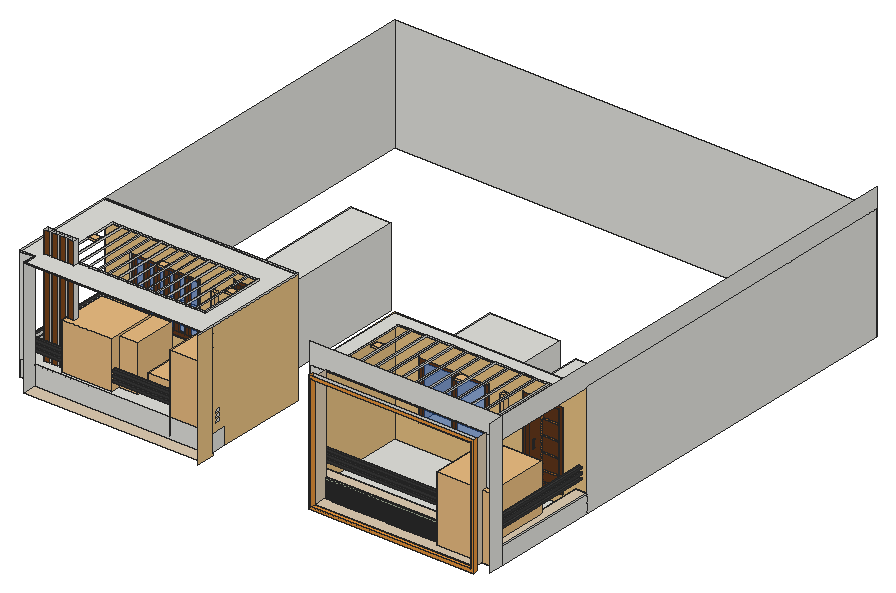
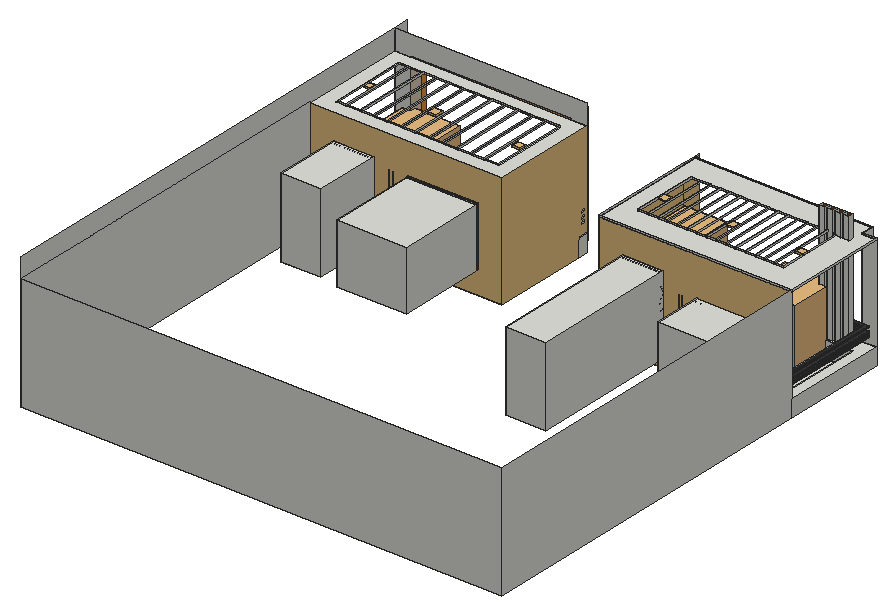
# SketchUp Ruby script. Lengths in inches.
U = 1.inch
M = Sketchup.active_model
def pt(a) = Geom::Point3d.new(a.map { |v| v * U })
def face(e, loops, mat)
  f = e.add_face(loops[0].map { |a| pt(a) })
  loops[1..].each { |l| e.add_face(l.map { |a| pt(a) }).erase! }
  f.material = f.back_material = mat if mat
  f
end
# faces: each face lists its corners as indices into pts; further lists are holes
def faces(e, pts, list, mat = nil) = list.each { |f| face(e, (f[0].is_a?(Array) ? f : [f]).map { |l| l.map { |i| pts[i] } }, mat) }
# xy, xz, yz: faces in a plane at the given z, y or x. An outline is a flat list of corners, or four numbers for a rectangle; further outlines are holes
def ring(l) = l.size == 4 ? [[l[0], l[1]], [l[2], l[1]], [l[2], l[3]], [l[0], l[3]]] : l.each_slice(2).to_a
def flat(e, list, mat, &to3) = list.each { |f| face(e, (f[0].is_a?(Array) ? f : [f]).map { |l| ring(l).map { |u, v| to3.(u, v) } }, mat) }
def xy(e, z, list, mat = nil) = flat(e, list, mat) { |x, y| [x, y, z] }
def xz(e, y, list, mat = nil) = flat(e, list, mat) { |x, z| [x, y, z] }
def yz(e, x, list, mat = nil) = flat(e, list, mat) { |y, z| [x, y, z] }
def lines(e, pts, list) = list.each { |a, b| e.add_line(pt(pts[a]), pt(pts[b])) }
# prism: a flat outline (further loops are holes) pulled along v
def prism(e, loops, v, mat = nil)
  f = face(e, loops, mat); d = Geom::Vector3d.new(v.map { |x| x * U })
  f.pushpull(f.normal.samedirection?(d) ? d.length : -d.length)
end
def box(e, o, s, mat = nil) = prism(e, [[o, [o[0] + s[0], o[1], o[2]], [o[0] + s[0], o[1] + s[1], o[2]], [o[0], o[1] + s[1], o[2]]]], [0, 0, s[2]], mat)
def at(x, y, z, deg = 0) = Geom::Transformation.translation(pt([x, y, z])) * Geom::Transformation.rotation(ORIGIN, Z_AXIS, deg.degrees)
def axes(o, x, y, z) = Geom::Transformation.new([*x, 0, *y, 0, *z, 0, *pt(o).to_a, 1])
def part(name) = M.definitions.add(name)
# library, detail: a bought-in or finely detailed component or shape, given as its bounding box
def library(name, o, s) = part(name).tap { |d| box(d.entities, o, s) }
def detail(e, o, s) = box(e.add_group.entities, o, s)
def put(e, d, t, mat = nil) = e.add_instance(d, t).tap { |i| i.material = mat if mat }
def group(e, t, mat = nil) = e.add_group.tap { |g| g.transformation = t; g.material = mat if mat }.entities
root = M.entities
M.materials.add("Generic\#1").color = [121, 68, 27]
M.materials.add("Generic\#4").color = [232, 149, 60]
M.materials.add("Generic\#5").color = [233, 194, 132]
M.materials.add("Generic\#6").color = [223, 205, 179]
M.materials.add("Generic\#8").color = [168, 180, 155]
M.materials.add("[Color M05]").color = [114, 114, 114]
M.materials.add("[Color M07]").color = [58, 58, 58]
M.materials.add("[Translucent Glass Blue]").color = [28, 83, 181]
M.materials["[Translucent Glass Blue]"].alpha = 0.5
M.materials.add("[Wood Bamboo]").color = [177, 105, 43]
M.materials.add("[Wood Cherry Original]").color = [96, 54, 26]
c1 = library("Plante 4",[-1.67,-6.5,0],[37.31,31.95,64.42])
c2 = library("Group_2",[-1.28,-0.39,0],[21.22,20.51,48.44])
c3 = library("Group3\#1",[-238.15,54.18,0],[46.4,43.96,56.68])
c4 = library("Plant",[-27.84,-31.84,-1.26],[68.28,70.82,154.38])
c5 = library("Raised potted plant",[1.65,0,0],[13.63,13.63,20.73])
c6 = library("Plant+2 (1)",[-9.13,-9.52,0],[51.76,51.77,66.88])
c7 = part("Group\#12")
xy(c7.entities,17.5625,[[0,0,2,2]])
xz(c7.entities,0,[[0,0,2,17.5625]])
yz(c7.entities,0,[[0,0,2,17.5625]])
yz(c7.entities,2,[[0,0,2,17.5625]])
c8 = part("Group\#5")
xy(c8.entities,0,[[0,0,41.8125,3.4375]],"[Wood Cherry Original]")
xy(c8.entities,3.53,[[3.53,0,38.28,3.4375]],"[Wood Cherry Original]")
xy(c8.entities,31.39,[[9.28,1.32,9.97,3.4375]])
xy(c8.entities,32.05,[[9.29,1.98,9.98,3.4375]],"[Color M05]")
xy(c8.entities,39.77,[[9.29,1.98,9.98,3.4375]])
xy(c8.entities,40.43,[[9.28,1.32,9.97,3.4375]],"[Color M05]")
xy(c8.entities,79.47,[[3.53,0,38.28,3.4375]],"[Wood Cherry Original]")
xy(c8.entities,83,[[0,0,41.8125,3.4375]],"[Wood Cherry Original]")
xz(c8.entities,0,[[[0,0,41.8125,83],[3.53,3.53,38.28,79.47]]],"[Wood Cherry Original]")
xz(c8.entities,1.32,[[9.28,31.39,9.97,40.43]],"[Color M05]")
xz(c8.entities,1.98,[[9.29,32.05,9.98,39.77]],"[Color M05]")
xz(c8.entities,3.4375,[[9.29,39.77,9.28,40.43,9.97,40.43,9.98,39.77]])
xz(c8.entities,3.4375,[[16.22,3.53,17.74,3.53,17.74,13.29,38.28,13.29,38.28,15.09,17.74,15.09,17.74,29.41,38.28,29.41,38.28,31.22,17.74,31.22,17.74,45.54,38.28,45.54,38.28,47.34,17.74,47.34,17.74,61.66,38.28,61.66,38.28,63.47,17.74,63.47,17.74,79.47,16.22,79.47]],"[Wood Bamboo]")
xz(c8.entities,3.4375,[[[0,0,41.8125,83],[3.53,3.53,38.28,79.47]],[[3.53,3.53,16.22,79.47],[9.29,39.77,9.28,40.43,9.97,40.43,9.98,39.77],[9.28,31.39,9.29,32.05,9.98,32.05,9.97,31.39]],[17.74,3.53,38.28,13.29],[17.74,15.09,38.28,29.41],[17.74,31.22,38.28,45.54],
  [17.74,47.34,38.28,61.66],[17.74,63.47,38.28,79.47]],"[Wood Cherry Original]")
yz(c8.entities,0,[[0,0,3.4375,83]],"[Wood Cherry Original]")
yz(c8.entities,3.53,[[0,3.53,3.4375,79.47]],"[Wood Cherry Original]")
yz(c8.entities,38.28,[[0,3.53,3.4375,79.47]],"[Wood Cherry Original]")
yz(c8.entities,41.8125,[[0,0,3.4375,83]],"[Wood Cherry Original]")
p = [[9.28,1.32,40.43],[9.29,1.98,39.77],[9.29,1.98,32.05],[9.28,1.32,31.39],[9.29,3.4375,32.05],[9.28,3.4375,31.39],
  [9.98,1.98,39.77],[9.97,1.32,40.43],[9.97,1.32,31.39],[9.98,1.98,32.05],[9.97,3.4375,31.39],[9.98,3.4375,32.05],
  [9.28,3.4375,40.43],[9.29,3.4375,39.77],[9.98,3.4375,39.77],[9.97,3.4375,40.43],[9.625,3.4375,40.13],[9.625,1.625,40.13],
  [9.625,1.625,31.69],[9.625,3.4375,31.69]]
faces(c8.entities,p,[[0,1,2,3],[3,2,4,5],[6,7,8,9],[9,8,10,11],[12,13,1,0],[14,15,7,6]],"[Color M05]")
lines(c8.entities,p,[[16,17],[18,19],[17,18]])
c9 = part("Group\#3")
xy(c9.entities,0,[[0,0,81.86,2.5]],"[Wood Cherry Original]")
xy(c9.entities,4.12,[[4.12,0,13.68,2.5],[13.68,0,18.93,2.5],[18.93,0,25.68,2.5],[25.68,0,30.93,2.5],[30.93,0,37.68,2.5],
  [37.68,0,42.93,2.5],[42.93,0,49.68,2.5],[49.68,0,54.93,2.5],[54.93,0,61.68,2.5],[61.68,0,66.93,2.5],
  [66.93,0,77.74,2.5]],"[Wood Cherry Original]")
xy(c9.entities,66.49,[[4.12,0,13.68,2.5],[13.68,0,18.93,2.5],[18.93,0,25.68,2.5],[25.68,0,30.93,2.5],[30.93,0,37.68,2.5],
  [37.68,0,42.93,2.5],[42.93,0,49.68,2.5],[49.68,0,54.93,2.5],[54.93,0,61.68,2.5],[61.68,0,66.93,2.5],
  [66.93,0,77.74,2.5]],"[Wood Cherry Original]")
xy(c9.entities,70.61,[[0,0,81.86,2.5]],"[Wood Cherry Original]")
xz(c9.entities,0,[[[0,0,81.86,70.61],[4.12,4.12,77.74,66.49]],[13.68,4.12,18.93,66.49],[25.68,4.12,30.93,66.49],[37.68,4.12,42.93,66.49],[49.68,4.12,54.93,66.49],
  [61.68,4.12,66.93,66.49]],"[Wood Cherry Original]")
xz(c9.entities,2.5,[[4.12,4.12,13.68,66.49],[18.93,4.12,25.68,66.49],[30.93,4.12,37.68,66.49],[42.93,4.12,49.68,66.49],[54.93,4.12,61.68,66.49],
  [66.93,4.12,77.74,66.49]],"[Translucent Glass Blue]")
xz(c9.entities,2.5,[[[0,0,81.86,70.61],[4.12,4.12,77.74,66.49]]],"[Wood Cherry Original]")
yz(c9.entities,0,[[0,0,2.5,70.61]],"[Wood Cherry Original]")
yz(c9.entities,4.12,[[0,4.12,2.5,66.49]],"[Wood Cherry Original]")
yz(c9.entities,13.68,[[0,4.12,2.5,66.49]],"[Wood Cherry Original]")
yz(c9.entities,18.93,[[0,4.12,2.5,66.49]],"[Wood Cherry Original]")
yz(c9.entities,25.68,[[0,4.12,2.5,66.49]],"[Wood Cherry Original]")
yz(c9.entities,30.93,[[0,4.12,2.5,66.49]],"[Wood Cherry Original]")
yz(c9.entities,37.68,[[0,4.12,2.5,66.49]],"[Wood Cherry Original]")
yz(c9.entities,42.93,[[0,4.12,2.5,66.49]],"[Wood Cherry Original]")
yz(c9.entities,49.68,[[0,4.12,2.5,66.49]],"[Wood Cherry Original]")
yz(c9.entities,54.93,[[0,4.12,2.5,66.49]],"[Wood Cherry Original]")
yz(c9.entities,61.68,[[0,4.12,2.5,66.49]],"[Wood Cherry Original]")
yz(c9.entities,66.93,[[0,4.12,2.5,66.49]],"[Wood Cherry Original]")
yz(c9.entities,77.74,[[0,4.12,2.5,66.49]],"[Wood Cherry Original]")
yz(c9.entities,81.86,[[0,0,2.5,70.61]],"[Wood Cherry Original]")
c10 = part("Group\#4")
xy(c10.entities,0,[[0,0,73.625,2.0625]],"[Wood Cherry Original]")
xy(c10.entities,3.98,[[35.0625,0,38.75,2.0625]])
xy(c10.entities,3.98,[[3.98,0,35.0625,2.0625],[38.75,0,69.64,2.0625]],"[Wood Cherry Original]")
xy(c10.entities,58.39,[[35.0625,0,38.75,2.0625]])
xy(c10.entities,58.39,[[3.98,0,35.0625,2.0625],[38.75,0,69.64,2.0625]],"[Wood Cherry Original]")
xy(c10.entities,62.375,[[0,0,73.625,2.0625]],"[Wood Cherry Original]")
xz(c10.entities,0,[[[0,0,73.625,62.375],[3.98,3.98,69.64,58.39]],[35.0625,3.98,38.75,58.39]],"[Wood Cherry Original]")
xz(c10.entities,2.0625,[[[0,0,73.625,62.375],[3.98,3.98,69.64,58.39]]])
xz(c10.entities,2.0625,[[3.98,3.98,35.0625,58.39],[38.75,3.98,69.64,58.39]],"[Translucent Glass Blue]")
yz(c10.entities,0,[[0,0,2.0625,62.375]],"[Wood Cherry Original]")
yz(c10.entities,3.98,[[0,3.98,2.0625,58.39]],"[Wood Cherry Original]")
yz(c10.entities,35.0625,[[0,3.98,2.0625,58.39]],"[Wood Cherry Original]")
yz(c10.entities,38.75,[[0,3.98,2.0625,58.39]],"[Wood Cherry Original]")
yz(c10.entities,69.64,[[0,3.98,2.0625,58.39]],"[Wood Cherry Original]")
yz(c10.entities,73.625,[[0,0,2.0625,62.375]],"[Wood Cherry Original]")
c11 = library("Lamp Wall Outdoor 94-02",[-1.89,-4.65,-3.17],[3.78,4.65,6.35])
c12 = library("Tlon Light 450 Ceiling 152 006",[-8.86,-8.86,-3.78],[17.72,17.72,3.56])
xy(root,278.625,[[321.31,34.75,494.1875,39.375]],"Generic\#4")
xy(root,278.75,[[17.125,41,204.09,54.5625]],"Generic\#6")
xy(root,281.75,[[306.09,54.5625,306.09,65.5625,496.1875,65.5625,496.1875,166.1875,507.875,166.1875,507.875,54.5625],[306.09,65.5625,496.1875,166.1875],[13.4375,71.3125,204.09,166.1875]])
xy(root,281.75,[[323.78,34.75,491.8125,39.375]],"Generic\#4")
xy(root,281.75,[[323.78,39.375,491.8125,54.5625]],"Generic\#6")
xy(root,289.8,[[137.36,166.1875,179.17,320.375]])
xy(root,290.68,[[440.99,166.1875,482.8,235.75]])
xy(root,297.03,[[27.78,166.1875,101.4,217.3125]])
xy(root,299.3125,[[323.78,52.5625,325.78,54.5625],[325.78,52.5625,491.8125,54.5625],[[2.3125,54.5625,204.09,54.5625,204.09,71.3125,13.4375,71.3125,13.4375,166.1875,2.3125,166.1875],[19.41,64.07,25.6,69.2],[27.85,64.07,34.03,69.2],[36.28,64.07,42.47,69.2],[44.72,64.07,50.91,69.2]],[306.09,54.5625,306.09,65.5625,496.1875,65.5625,496.1875,166.1875,507.875,166.1875,507.875,54.5625]])
xy(root,301.3125,[[306.09,54.5625,507.875,54.5625,507.875,166.1875,496.1875,166.1875,496.1875,65.5625,306.09,65.5625]],"Generic\#6")
xy(root,301.3125,[[323.78,52.5625,491.8125,54.5625]],"Generic\#8")
xy(root,305.15,[[331.4,166.1875,405.03,260.1875]])
xy(root,308.18,[[6.99,59.18,6.99,166.1875,10.24,166.1875,10.24,62.43,204.09,62.43,204.09,59.18]],"[Color M07]")
xy(root,310.93,[[6.99,59.18,204.09,59.18,204.09,62.43,10.24,62.43,10.24,166.1875,6.99,166.1875]],"[Color M07]")
xy(root,311.86,[[306.09,58.82,306.09,61.82,500.27,61.82,500.27,166.1875,503.27,166.1875,503.27,58.82]],"[Color M07]")
xy(root,312.62,[[6.99,59.18,6.99,166.1875,10.24,166.1875,10.24,62.43,204.09,62.43,204.09,59.18]],"[Color M07]")
xy(root,314.42,[[306.09,58.82,503.27,58.82,503.27,166.1875,500.27,166.1875,500.27,61.82,306.09,61.82]],"[Color M07]")
xy(root,315.37,[[6.99,59.18,204.09,59.18,204.09,62.43,10.24,62.43,10.24,166.1875,6.99,166.1875]],"[Color M07]")
xy(root,316.8,[[306.09,58.82,306.09,61.82,500.27,61.82,500.27,166.1875,503.27,166.1875,503.27,58.82]],"[Color M07]")
xy(root,317.37,[[6.99,59.18,6.99,166.1875,10.24,166.1875,10.24,62.43,204.09,62.43,204.09,59.18]],"[Color M07]")
xy(root,319.36,[[306.09,58.82,503.27,58.82,503.27,166.1875,500.27,166.1875,500.27,61.82,306.09,61.82]],"[Color M07]")
xy(root,320.12,[[6.99,59.18,204.09,59.18,204.09,62.43,10.24,62.43,10.24,166.1875,6.99,166.1875]],"[Color M07]")
xy(root,322.36,[[306.09,58.82,306.09,61.82,500.27,61.82,500.27,166.1875,503.27,166.1875,503.27,58.82]],"[Color M07]")
xy(root,324.92,[[306.09,58.82,503.27,58.82,503.27,166.1875,500.27,166.1875,500.27,61.82,306.09,61.82]],"[Color M07]")
xy(root,359.4,[[27.78,166.1875,101.4,217.3125]])
xy(root,367.53,[[331.4,166.1875,405.03,260.1875]])
xy(root,372.8,[[137.36,166.1875,179.17,320.375]])
xy(root,373.68,[[440.99,166.1875,482.8,235.75]])
xy(root,400.3125,[[[17.125,41,17.125,54.5625,2.3125,54.5625,2.3125,166.1875,204.09,166.1875,204.09,41],[32.72,68.9375,185.53,138.25]],[41.97,68.9375,42.91,138.25],[52.16,68.9375,53.09,138.25],[62.34,68.9375,63.28,138.25],[72.53,68.9375,73.47,138.25],
  [82.72,68.9375,83.66,138.25],[92.91,68.9375,93.84,138.25],[103.09,68.9375,104.03,138.25],[113.28,68.9375,114.22,138.25],[123.47,68.9375,124.41,138.25],
  [133.66,68.9375,134.59,138.25],[143.84,68.9375,144.78,138.25],[154.03,68.9375,154.97,138.25],[164.22,68.9375,165.16,138.25],[174.41,68.9375,175.34,138.25],
  [184.59,68.9375,185.53,138.25]])
xy(root,400.625,[[[306.09,54.5625,507.875,166.1875],[321.03,69.49,492.94,151.25]],[321.03,69.49,323.03,151.25],[335.53,69.49,337.53,151.25],[350.03,69.49,352.03,151.25],[364.53,69.49,366.53,151.25],
  [379.03,69.49,381.03,151.25],[393.53,69.49,395.53,151.25],[408.03,69.49,410.03,151.25],[422.53,69.49,424.53,151.25],[437.03,69.49,439.03,151.25],
  [451.53,69.49,453.53,151.25],[466.03,69.49,468.03,151.25],[480.53,69.49,482.53,151.25],[490.94,69.49,492.94,151.25]])
xz(root,34.75,[[[321.31,278.625,494.1875,404.6875],[323.78,281.75,491.8125,401.75]]],"Generic\#4")
xz(root,39.375,[[[321.31,278.625,494.1875,404.6875],[323.78,281.75,491.8125,401.75]]])
xz(root,41,[[17.125,400.3125,204.09,401.75]],"Generic\#4")
xz(root,52.5625,[[323.78,299.3125,491.8125,301.3125]],"Generic\#8")
xz(root,54.5625,[[17.125,278.75,204.09,299.3125],[2.3125,281.75,17.125,299.3125],[306.09,281.75,323.78,299.3125],[323.78,281.75,325.78,299.3125],[325.78,281.75,491.8125,299.3125],
  [491.8125,281.75,507.875,299.3125],[2.3125,299.3125,17.125,400.3125],[306.09,299.3125,323.78,301.3125],[323.78,299.3125,491.8125,301.3125],[491.8125,299.3125,507.875,301.3125],
  [306.09,301.3125,323.78,400.625],[491.8125,301.3125,507.875,400.625],[2.3125,400.3125,17.125,401.75],[306.09,400.625,306.09,422.625,507.875,422.625,507.875,400.625,491.8125,400.625,491.8125,401.75,323.78,401.75,323.78,400.625]])
xz(root,54.5625,[[323.78,400.625,491.8125,401.75]],"Generic\#4")
xz(root,58.82,[[306.09,311.86,503.27,314.42],[306.09,316.8,503.27,319.36],[306.09,322.36,503.27,324.92]],"[Color M07]")
xz(root,59.18,[[6.99,308.18,204.09,310.93],[6.99,312.62,204.09,315.37],[6.99,317.37,204.09,320.12]],"[Color M07]")
xz(root,61.82,[[306.09,311.86,500.27,314.42],[306.09,316.8,500.27,319.36],[306.09,322.36,500.27,324.92]],"[Color M07]")
xz(root,62.43,[[10.24,308.18,204.09,310.93],[10.24,312.62,204.09,315.37],[10.24,317.37,204.09,320.12]],"[Color M07]")
xz(root,64.07,[[19.41,299.3125,25.6,422.625],[27.85,299.3125,34.03,422.625],[36.28,299.3125,42.47,422.625],[44.72,299.3125,50.91,422.625]],"Generic\#1")
xz(root,65.5625,[[306.09,281.75,496.1875,299.3125],[306.09,299.3125,496.1875,301.3125]])
xz(root,68.9375,[[32.72,400.3125,41.97,401.75],[41.97,400.3125,42.91,401.75],[42.91,400.3125,52.16,401.75],[52.16,400.3125,53.09,401.75],[53.09,400.3125,62.34,401.75],
  [62.34,400.3125,63.28,401.75],[63.28,400.3125,72.53,401.75],[72.53,400.3125,73.47,401.75],[73.47,400.3125,82.72,401.75],[82.72,400.3125,83.66,401.75],
  [83.66,400.3125,92.91,401.75],[92.91,400.3125,93.84,401.75],[93.84,400.3125,103.09,401.75],[103.09,400.3125,104.03,401.75],[104.03,400.3125,113.28,401.75],
  [113.28,400.3125,114.22,401.75],[114.22,400.3125,123.47,401.75],[123.47,400.3125,124.41,401.75],[124.41,400.3125,133.66,401.75],[133.66,400.3125,134.59,401.75],
  [134.59,400.3125,143.84,401.75],[143.84,400.3125,144.78,401.75],[144.78,400.3125,154.03,401.75],[154.03,400.3125,154.97,401.75],[154.97,400.3125,164.22,401.75],
  [164.22,400.3125,165.16,401.75],[165.16,400.3125,174.41,401.75],[174.41,400.3125,175.34,401.75],[175.34,400.3125,184.59,401.75],[184.59,400.3125,185.53,401.75]])
xz(root,69.2,[[19.41,299.3125,25.6,422.625],[27.85,299.3125,34.03,422.625],[36.28,299.3125,42.47,422.625],[44.72,299.3125,50.91,422.625]])
xz(root,69.49,[[323.03,400.625,323.78,401.75],[323.78,400.625,335.53,401.75],[337.53,400.625,350.03,401.75],[352.03,400.625,364.53,401.75],[366.53,400.625,379.03,401.75],
  [381.03,400.625,393.53,401.75],[395.53,400.625,408.03,401.75],[410.03,400.625,422.53,401.75],[424.53,400.625,437.03,401.75],[439.03,400.625,451.53,401.75],
  [453.53,400.625,466.03,401.75],[468.03,400.625,480.53,401.75],[482.53,400.625,490.94,401.75]])
xz(root,71.3125,[[13.4375,281.75,204.09,299.3125]])
xz(root,138.25,[[32.72,400.3125,41.97,401.75],[41.97,400.3125,42.91,401.75],[42.91,400.3125,52.16,401.75],[52.16,400.3125,53.09,401.75],[53.09,400.3125,62.34,401.75],
  [62.34,400.3125,63.28,401.75],[63.28,400.3125,72.53,401.75],[72.53,400.3125,73.47,401.75],[73.47,400.3125,82.72,401.75],[82.72,400.3125,83.66,401.75],
  [83.66,400.3125,92.91,401.75],[92.91,400.3125,93.84,401.75],[93.84,400.3125,103.09,401.75],[103.09,400.3125,104.03,401.75],[104.03,400.3125,113.28,401.75],
  [113.28,400.3125,114.22,401.75],[114.22,400.3125,123.47,401.75],[123.47,400.3125,124.41,401.75],[124.41,400.3125,133.66,401.75],[133.66,400.3125,134.59,401.75],
  [134.59,400.3125,143.84,401.75],[143.84,400.3125,144.78,401.75],[144.78,400.3125,154.03,401.75],[154.03,400.3125,154.97,401.75],[154.97,400.3125,164.22,401.75],
  [164.22,400.3125,165.16,401.75],[165.16,400.3125,174.41,401.75],[174.41,400.3125,175.34,401.75],[175.34,400.3125,184.59,401.75],[184.59,400.3125,185.53,401.75]])
xz(root,151.25,[[323.03,400.625,335.53,401.75],[337.53,400.625,350.03,401.75],[352.03,400.625,364.53,401.75],[366.53,400.625,379.03,401.75],[381.03,400.625,393.53,401.75],
  [395.53,400.625,408.03,401.75],[410.03,400.625,422.53,401.75],[424.53,400.625,437.03,401.75],[439.03,400.625,451.53,401.75],[453.53,400.625,466.03,401.75],
  [468.03,400.625,480.53,401.75],[482.53,400.625,490.94,401.75]])
xz(root,166.1875,[[496.1875,299.3125,507.875,301.3125],[2.3125,400.3125,204.09,401.75]])
xz(root,166.1875,[[[13.4375,281.75,204.09,281.75,204.09,400.3125,2.3125,400.3125,2.3125,299.3125,13.4375,299.3125],[27.78,297.03,101.4,359.4],[137.36,289.8,179.17,372.8],[6.99,317.37,10.24,320.12],[6.99,312.62,10.24,315.37],[6.99,308.18,10.24,310.93]],[[306.09,281.75,496.1875,281.75,496.1875,301.3125,507.875,301.3125,507.875,400.625,306.09,400.625],[331.4,305.15,405.03,367.53],[440.99,290.68,482.8,373.68],[500.27,311.86,503.27,314.42],[500.27,316.8,503.27,319.36],[500.27,322.36,503.27,324.92]]],"Generic\#5")
xz(root,217.3125,[[27.78,297.03,101.4,359.4]])
xz(root,235.75,[[440.99,290.68,482.8,373.68]])
xz(root,260.1875,[[331.4,305.15,405.03,367.53]])
xz(root,320.375,[[137.36,289.8,179.17,372.8]])
xz(root,546.8125,[[2.3125,281.75,507.875,401.75]])
yz(root,2.3125,[[54.5625,281.75,166.1875,299.3125],[166.1875,281.75,546.8125,401.75],[54.5625,400.3125,166.1875,401.75]])
yz(root,6.99,[[59.18,308.18,166.1875,310.93],[59.18,312.62,166.1875,315.37],[59.18,317.37,166.1875,320.12]],"[Color M07]")
yz(root,10.24,[[62.43,308.18,166.1875,310.93],[62.43,312.62,166.1875,315.37],[62.43,317.37,166.1875,320.12]])
yz(root,13.4375,[[71.3125,281.75,166.1875,299.3125]])
yz(root,17.125,[[41,278.75,54.5625,400.3125],[41,400.3125,54.5625,401.75]])
yz(root,19.41,[[64.07,299.3125,69.2,422.625]])
yz(root,25.6,[[64.07,299.3125,69.2,422.625]])
yz(root,27.78,[[166.1875,297.03,217.3125,359.4]])
yz(root,27.85,[[64.07,299.3125,69.2,422.625]])
yz(root,32.72,[[68.9375,400.3125,138.25,401.75]])
yz(root,34.03,[[64.07,299.3125,69.2,422.625]])
yz(root,36.28,[[64.07,299.3125,69.2,422.625]])
yz(root,41.97,[[68.9375,400.3125,138.25,401.75]])
yz(root,42.47,[[64.07,299.3125,69.2,422.625]])
yz(root,42.91,[[68.9375,400.3125,138.25,401.75]])
yz(root,44.72,[[64.07,299.3125,69.2,422.625]])
yz(root,50.91,[[64.07,299.3125,69.2,422.625]])
yz(root,52.16,[[68.9375,400.3125,138.25,401.75]])
yz(root,53.09,[[68.9375,400.3125,138.25,401.75]])
yz(root,62.34,[[68.9375,400.3125,138.25,401.75]])
yz(root,63.28,[[68.9375,400.3125,138.25,401.75]])
yz(root,72.53,[[68.9375,400.3125,138.25,401.75]])
yz(root,73.47,[[68.9375,400.3125,138.25,401.75]])
yz(root,82.72,[[68.9375,400.3125,138.25,401.75]])
yz(root,83.66,[[68.9375,400.3125,138.25,401.75]])
yz(root,92.91,[[68.9375,400.3125,138.25,401.75]])
yz(root,93.84,[[68.9375,400.3125,138.25,401.75]])
yz(root,101.4,[[166.1875,297.03,217.3125,359.4]])
yz(root,103.09,[[68.9375,400.3125,138.25,401.75]])
yz(root,104.03,[[68.9375,400.3125,138.25,401.75]])
yz(root,113.28,[[68.9375,400.3125,138.25,401.75]])
yz(root,114.22,[[68.9375,400.3125,138.25,401.75]])
yz(root,123.47,[[68.9375,400.3125,138.25,401.75]])
yz(root,124.41,[[68.9375,400.3125,138.25,401.75]])
yz(root,133.66,[[68.9375,400.3125,138.25,401.75]])
yz(root,134.59,[[68.9375,400.3125,138.25,401.75]])
yz(root,137.36,[[166.1875,289.8,320.375,372.8]])
yz(root,143.84,[[68.9375,400.3125,138.25,401.75]])
yz(root,144.78,[[68.9375,400.3125,138.25,401.75]])
yz(root,154.03,[[68.9375,400.3125,138.25,401.75]])
yz(root,154.97,[[68.9375,400.3125,138.25,401.75]])
yz(root,164.22,[[68.9375,400.3125,138.25,401.75]])
yz(root,165.16,[[68.9375,400.3125,138.25,401.75]])
yz(root,174.41,[[68.9375,400.3125,138.25,401.75]])
yz(root,175.34,[[68.9375,400.3125,138.25,401.75]])
yz(root,179.17,[[166.1875,289.8,320.375,372.8]])
yz(root,184.59,[[68.9375,400.3125,138.25,401.75]])
yz(root,185.53,[[68.9375,400.3125,138.25,401.75]])
yz(root,204.09,[[54.5625,281.75,71.3125,299.3125],[59.18,308.18,62.43,310.93],[59.18,312.62,62.43,315.37],[59.18,317.37,62.43,320.12],[35.5625,400.3125,41,401.75],
  [41,400.3125,54.5625,401.75],[54.5625,400.3125,166.1875,401.75]])
yz(root,204.09,[[35.5625,278.75,54.5625,400.3125],[[71.3125,281.75,71.3125,299.3125,54.5625,299.3125,54.5625,400.3125,166.1875,400.3125,166.1875,281.75],[59.18,317.37,62.43,320.12],[59.18,312.62,62.43,315.37],[59.18,308.18,62.43,310.93]]],"Generic\#5")
yz(root,306.09,[[54.5625,281.75,65.5625,299.3125],[54.5625,299.3125,65.5625,301.3125],[58.82,311.86,61.82,314.42],[58.82,316.8,61.82,319.36],[58.82,322.36,61.82,324.92]])
yz(root,306.09,[[[65.5625,281.75,166.1875,281.75,166.1875,400.625,54.5625,400.625,54.5625,301.3125,65.5625,301.3125],[58.82,322.36,61.82,324.92],[58.82,316.8,61.82,319.36],[58.82,311.86,61.82,314.42]]],"Generic\#5")
yz(root,321.31,[[34.75,278.625,39.375,404.6875]],"Generic\#4")
yz(root,323.03,[[69.49,400.625,151.25,401.75]])
yz(root,323.78,[[52.5625,299.3125,54.5625,301.3125]])
yz(root,323.78,[[34.75,281.75,39.375,401.75]],"Generic\#4")
yz(root,323.78,[[39.375,281.75,54.5625,281.75,54.5625,299.3125,52.5625,299.3125,52.5625,301.3125,54.5625,301.3125,54.5625,401.75,39.375,401.75]],"Generic\#6")
yz(root,331.4,[[166.1875,305.15,260.1875,367.53]])
yz(root,335.53,[[69.49,400.625,151.25,401.75]])
yz(root,337.53,[[69.49,400.625,151.25,401.75]])
yz(root,350.03,[[69.49,400.625,151.25,401.75]])
yz(root,352.03,[[69.49,400.625,151.25,401.75]])
yz(root,364.53,[[69.49,400.625,151.25,401.75]])
yz(root,366.53,[[69.49,400.625,151.25,401.75]])
yz(root,379.03,[[69.49,400.625,151.25,401.75]])
yz(root,381.03,[[69.49,400.625,151.25,401.75]])
yz(root,393.53,[[69.49,400.625,151.25,401.75]])
yz(root,395.53,[[69.49,400.625,151.25,401.75]])
yz(root,405.03,[[166.1875,305.15,260.1875,367.53]])
yz(root,408.03,[[69.49,400.625,151.25,401.75]])
yz(root,410.03,[[69.49,400.625,151.25,401.75]])
yz(root,422.53,[[69.49,400.625,151.25,401.75]])
yz(root,424.53,[[69.49,400.625,151.25,401.75]])
yz(root,437.03,[[69.49,400.625,151.25,401.75]])
yz(root,439.03,[[69.49,400.625,151.25,401.75]])
yz(root,440.99,[[166.1875,290.68,235.75,373.68]])
yz(root,451.53,[[69.49,400.625,151.25,401.75]])
yz(root,453.53,[[69.49,400.625,151.25,401.75]])
yz(root,466.03,[[69.49,400.625,151.25,401.75]])
yz(root,468.03,[[69.49,400.625,151.25,401.75]])
yz(root,480.53,[[69.49,400.625,151.25,401.75]])
yz(root,482.53,[[69.49,400.625,151.25,401.75]])
yz(root,482.8,[[166.1875,290.68,235.75,373.68]])
yz(root,490.94,[[69.49,400.625,151.25,401.75]])
yz(root,491.8125,[[52.5625,299.3125,54.5625,301.3125]])
yz(root,491.8125,[[34.75,281.75,39.375,401.75]],"Generic\#4")
yz(root,491.8125,[[39.375,281.75,39.375,401.75,54.5625,401.75,54.5625,301.3125,52.5625,301.3125,52.5625,299.3125,54.5625,299.3125,54.5625,281.75]],"Generic\#6")
yz(root,494.1875,[[34.75,278.625,39.375,404.6875]],"Generic\#4")
yz(root,496.1875,[[65.5625,281.75,166.1875,299.3125],[65.5625,299.3125,166.1875,301.3125]])
yz(root,500.27,[[61.82,311.86,166.1875,314.42],[61.82,316.8,166.1875,319.36],[61.82,322.36,166.1875,324.92]],"[Color M07]")
yz(root,503.27,[[58.82,311.86,166.1875,314.42],[58.82,316.8,166.1875,319.36],[58.82,322.36,166.1875,324.92]],"[Color M07]")
yz(root,507.875,[[39.375,281.75,54.5625,422.625],[54.5625,281.75,166.1875,299.3125],[166.1875,281.75,546.8125,401.75],[54.5625,299.3125,166.1875,301.3125],[54.5625,400.625,166.1875,400.625,166.1875,401.75,546.8125,401.75,546.8125,422.625,54.5625,422.625]])
p = [[2.3125,166.1875,281.75],[13.4375,166.1875,281.75],[306.09,60.0625,313.0625],[502.03,60.0625,313.0625],[306.09,60.0625,318.375],[502.03,60.0625,318.375],
  [502.03,166.1875,318.375],[306.09,60.0625,323.6875],[502.03,60.0625,323.6875],[502.03,166.1875,323.6875],[502.03,166.1875,313.0625],[7.875,166.1875,309.3125],
  [7.875,60.0625,309.3125],[204.09,60.0625,309.3125],[7.875,166.1875,318.75],[7.875,60.0625,318.75],[204.09,60.0625,318.75],[7.875,166.1875,314],
  [7.875,60.0625,314],[204.09,60.0625,314],[325.78,54.5625,281.75],[325.78,52.5625,281.75]]
lines(root,p,[[0,1],[2,3],[4,5],[6,5],[7,8],[9,8],[10,3],[11,12],[13,12],[14,15],[16,15],[17,18],
  [19,18],[20,21]])
put(root,c1,axes([77.72,77.49,280.8],[1.03,0,0],[0,1.4214,0],[0,0,1.03]))
put(root,c2,axes([148.59,71.3125,281.75],[1.13,0,0],[0,1.356,0],[0,0,1.13]))
put(root,c3,axes([732.02,-35.31,281.75],[1.21,0,0],[0,1.5609,0],[0,0,1.21]))
put(root,c4,axes([177.11,75.72,282.4],[0.65,0,0],[0,0.65,0],[0,0,0.52]))
put(root,c5,axes([115.08,77.63,281.75],[1.7976,0,0],[0,1.98707,0],[0,0,1.68]))
put(root,c6,at(52.15,68.33,281.75))
put(root,c7,at(323.78,52.5625,281.75),"Generic\#1")
put(root,c7,at(326.59,52.5625,281.75),"Generic\#1")
put(root,c7,at(329.41,52.5625,281.75),"Generic\#1")
put(root,c7,at(332.22,52.5625,281.75),"Generic\#1")
put(root,c7,at(335.03,52.5625,281.75),"Generic\#1")
put(root,c7,at(337.84,52.5625,281.75),"Generic\#1")
put(root,c7,at(340.66,52.5625,281.75),"Generic\#1")
put(root,c7,at(343.47,52.5625,281.75),"Generic\#1")
put(root,c7,at(346.28,52.5625,281.75),"Generic\#1")
put(root,c7,at(349.09,52.5625,281.75),"Generic\#1")
put(root,c7,at(351.91,52.5625,281.75),"Generic\#1")
put(root,c7,at(354.72,52.5625,281.75),"Generic\#1")
put(root,c7,at(357.53,52.5625,281.75),"Generic\#1")
put(root,c7,at(360.34,52.5625,281.75),"Generic\#1")
put(root,c7,at(363.16,52.5625,281.75),"Generic\#1")
put(root,c7,at(365.97,52.5625,281.75),"Generic\#1")
put(root,c7,at(368.78,52.5625,281.75),"Generic\#1")
put(root,c7,at(371.59,52.5625,281.75),"Generic\#1")
put(root,c7,at(374.41,52.5625,281.75),"Generic\#1")
put(root,c7,at(377.22,52.5625,281.75),"Generic\#1")
put(root,c7,at(380.03,52.5625,281.75),"Generic\#1")
put(root,c7,at(382.84,52.5625,281.75),"Generic\#1")
put(root,c7,at(385.66,52.5625,281.75),"Generic\#1")
put(root,c7,at(388.47,52.5625,281.75),"Generic\#1")
put(root,c7,at(391.28,52.5625,281.75),"Generic\#1")
put(root,c7,at(394.09,52.5625,281.75),"Generic\#1")
put(root,c7,at(396.91,52.5625,281.75),"Generic\#1")
put(root,c7,at(399.72,52.5625,281.75),"Generic\#1")
put(root,c7,at(402.53,52.5625,281.75),"Generic\#1")
put(root,c7,at(405.34,52.5625,281.75),"Generic\#1")
put(root,c7,at(408.16,52.5625,281.75),"Generic\#1")
put(root,c7,at(410.97,52.5625,281.75),"Generic\#1")
put(root,c7,at(413.78,52.5625,281.75),"Generic\#1")
put(root,c7,at(416.59,52.5625,281.75),"Generic\#1")
put(root,c7,at(419.41,52.5625,281.75),"Generic\#1")
put(root,c7,at(422.22,52.5625,281.75),"Generic\#1")
put(root,c7,at(425.03,52.5625,281.75),"Generic\#1")
put(root,c7,at(427.84,52.5625,281.75),"Generic\#1")
put(root,c7,at(430.66,52.5625,281.75),"Generic\#1")
put(root,c7,at(433.47,52.5625,281.75),"Generic\#1")
put(root,c7,at(436.28,52.5625,281.75),"Generic\#1")
put(root,c7,at(439.09,52.5625,281.75),"Generic\#1")
put(root,c7,at(441.91,52.5625,281.75),"Generic\#1")
put(root,c7,at(444.72,52.5625,281.75),"Generic\#1")
put(root,c7,at(447.53,52.5625,281.75),"Generic\#1")
put(root,c7,at(450.34,52.5625,281.75),"Generic\#1")
put(root,c7,at(453.16,52.5625,281.75),"Generic\#1")
put(root,c7,at(455.97,52.5625,281.75),"Generic\#1")
put(root,c7,at(458.78,52.5625,281.75),"Generic\#1")
put(root,c7,at(461.59,52.5625,281.75),"Generic\#1")
put(root,c7,at(464.41,52.5625,281.75),"Generic\#1")
put(root,c7,at(467.22,52.5625,281.75),"Generic\#1")
put(root,c7,at(470.03,52.5625,281.75),"Generic\#1")
put(root,c7,at(472.84,52.5625,281.75),"Generic\#1")
put(root,c7,at(475.66,52.5625,281.75),"Generic\#1")
put(root,c7,at(478.47,52.5625,281.75),"Generic\#1")
put(root,c7,at(481.28,52.5625,281.75),"Generic\#1")
put(root,c7,at(484.09,52.5625,281.75),"Generic\#1")
put(root,c7,at(486.91,52.5625,281.75),"Generic\#1")
put(root,c7,at(489.72,52.5625,281.75),"Generic\#1")
put(root,c7,at(492.53,52.5625,281.75))
put(root,c7,at(495.34,52.5625,281.75))
put(root,c7,at(498.16,52.5625,281.75))
put(root,c7,at(500.97,52.5625,281.75))
put(root,c7,at(503.78,52.5625,281.75))
put(root,c8,at(440.99,166.1875,290.68))
put(root,c8,axes([137.36,166.1875,291.46],[1,0,0],[0,1,0],[0,0,0.98]))
put(root,c9,axes([27.78,168.92,296.78],[0.89936,0,0],[0,0.8633,0],[0,0,0.88057]))
put(root,c10,at(331.38,166.23,306.06))
put(root,c11,axes([118.9,166.1875,345.92],[1,0,0],[0,1,0],[0,0,3.19]))
put(root,c11,axes([422.9,166.1875,356.61],[1,0,0],[0,1,0],[0,0,3.19]))
put(root,c12,axes([329.84,114.67,401.24],[0.4425,0,0],[0,0.4425,0],[0,0,0.4425]))
put(root,c12,axes([418.02,114.39,401.86],[0.50887,0,0],[0,0.50887,0],[0,0,0.50887]))
put(root,c12,axes([487.43,113.89,401.48],[0.39692,0,0],[0,0.39692,0],[0,0,0.39692]))
put(root,c12,axes([36.69,109.39,402.01],[0.44852,0,0],[0,0.44852,0],[0,0,0.44852]))
put(root,c12,axes([108.63,109.39,402.01],[0.44852,0,0],[0,0.44852,0],[0,0,0.44852]))
put(root,c12,axes([180.62,109.39,402.01],[0.44852,0,0],[0,0.44852,0],[0,0,0.44852]))
